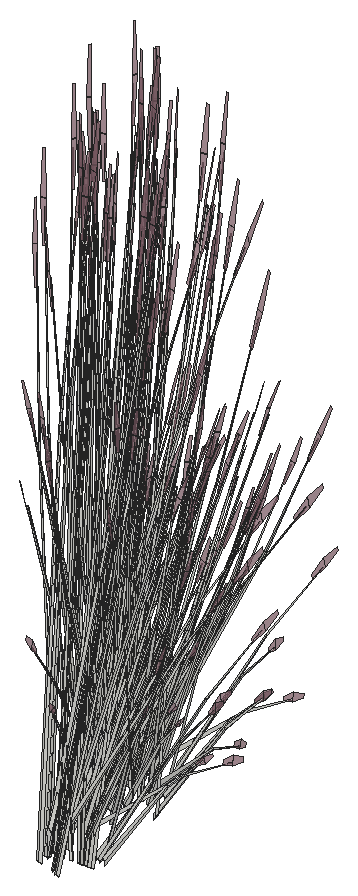
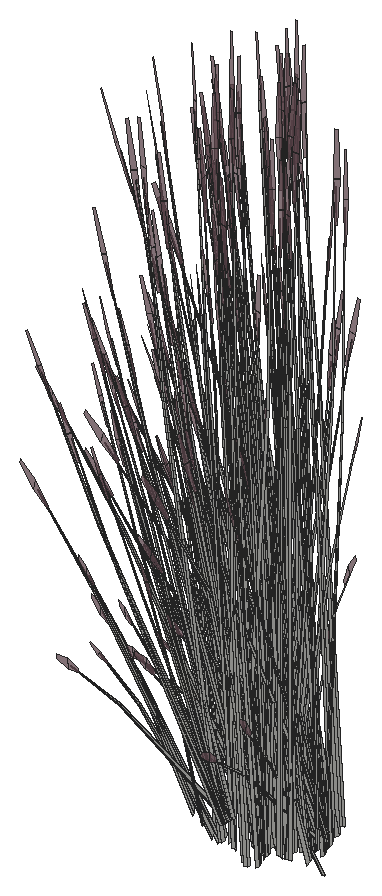
# SketchUp Ruby script. Lengths in inches.
U = 1.inch
M = Sketchup.active_model
def pt(a) = Geom::Point3d.new(a.map { |v| v * U })
def face(e, loops, mat)
  f = e.add_face(loops[0].map { |a| pt(a) })
  loops[1..].each { |l| e.add_face(l.map { |a| pt(a) }).erase! }
  f.material = f.back_material = mat if mat
  f
end
# faces: each face lists its corners as indices into pts; further lists are holes
def faces(e, pts, list, mat = nil) = list.each { |f| face(e, (f[0].is_a?(Array) ? f : [f]).map { |l| l.map { |i| pts[i] } }, mat) }
# xy, xz, yz: faces in a plane at the given z, y or x. An outline is a flat list of corners, or four numbers for a rectangle; further outlines are holes
def ring(l) = l.size == 4 ? [[l[0], l[1]], [l[2], l[1]], [l[2], l[3]], [l[0], l[3]]] : l.each_slice(2).to_a
def flat(e, list, mat, &to3) = list.each { |f| face(e, (f[0].is_a?(Array) ? f : [f]).map { |l| ring(l).map { |u, v| to3.(u, v) } }, mat) }
def xy(e, z, list, mat = nil) = flat(e, list, mat) { |x, y| [x, y, z] }
def xz(e, y, list, mat = nil) = flat(e, list, mat) { |x, z| [x, y, z] }
def yz(e, x, list, mat = nil) = flat(e, list, mat) { |y, z| [x, y, z] }
def lines(e, pts, list) = list.each { |a, b| e.add_line(pt(pts[a]), pt(pts[b])) }
# prism: a flat outline (further loops are holes) pulled along v
def prism(e, loops, v, mat = nil)
  f = face(e, loops, mat); d = Geom::Vector3d.new(v.map { |x| x * U })
  f.pushpull(f.normal.samedirection?(d) ? d.length : -d.length)
end
def box(e, o, s, mat = nil) = prism(e, [[o, [o[0] + s[0], o[1], o[2]], [o[0] + s[0], o[1] + s[1], o[2]], [o[0], o[1] + s[1], o[2]]]], [0, 0, s[2]], mat)
def at(x, y, z, deg = 0) = Geom::Transformation.translation(pt([x, y, z])) * Geom::Transformation.rotation(ORIGIN, Z_AXIS, deg.degrees)
def axes(o, x, y, z) = Geom::Transformation.new([*x, 0, *y, 0, *z, 0, *pt(o).to_a, 1])
def part(name) = M.definitions.add(name)
# library, detail: a bought-in or finely detailed component or shape, given as its bounding box
def library(name, o, s) = part(name).tap { |d| box(d.entities, o, s) }
def detail(e, o, s) = box(e.add_group.entities, o, s)
def put(e, d, t, mat = nil) = e.add_instance(d, t).tap { |i| i.material = mat if mat }
def group(e, t, mat = nil) = e.add_group.tap { |g| g.transformation = t; g.material = mat if mat }.entities
root = M.entities
M.materials.add("LightPink_Translucent").color = [144, 107, 117]
M.materials["LightPink_Translucent"].alpha = 0.75
c1 = part("blade")
p = [[2.15,0.21,22],[0,0.17,0],[0.09,0.45,0],[2.18,0.31,22],[2.29,0.31,22],[0.38,0.45,0],
  [2.48,0.24,33],[2.49,0.24,33],[2.48,0.22,33]]
faces(c1.entities,p,[[0,1,2,3],[4,5,2,3],[6,3,4,7],[8,0,3,6]])
c2 = part("seeds")
p = [[0.3,-0.1,1.38],[-0.01,-0.03,1.59],[-0.01,-0.03,0.03],[0.14,-0.07,-0.07],[0.29,-0.03,3],[0.15,0.01,3.11]]
faces(c2.entities,p,[[0,1,2,3],[1,0,4,5]],"LightPink_Translucent")
c3 = part("blade with seeds")
put(c3.entities,c1,at(0,0,0))
put(c3.entities,c2,axes([2.4,0.25,30.99],[1.5799,-0.05474,1.17369],[-0.12525,1.92788,0.29478],[-0.07173,-0.02425,1.56792]))
put(root,c3,axes([345.62,181.14,6.17],[-0.16657,0.22426,1.71376],[-0.69879,-0.4641,0.13857],[0.31524,-0.28926,0.73262]))
put(root,c3,axes([347.89,180.04,7],[-0.09085,0.04984,1.77383],[-0.89014,-0.16814,-0.16761],[-0.03222,-0.21748,0.31391]))
put(root,c3,axes([345.17,175.54,2.67],[0.90324,-0.43318,-0.29095],[0.60064,0.61207,-0.50002],[0.22285,0.06216,1.59708]))
put(root,c3,axes([348.76,176.68,4.53],[0.74348,0.18202,-0.35414],[-0.21685,0.53102,0.4572],[0.29933,-0.04869,0.87481]))
put(root,c3,axes([347.45,174.39,2.02],[0.83726,0.32623,-0.49651],[-0.50045,0.58498,0],[0.19069,0.0743,1.57504]))
put(root,c3,axes([345.86,176.25,2.21],[1.00089,0,0],[0,0.67548,0],[0,0,1.78407]))
put(root,c3,axes([345.16,179.42,5.06],[0.11476,0.38047,1.1486],[-0.63664,-0.21072,0.84392],[0.06851,-0.19481,0.25299]))
put(root,c3,axes([346.15,174.66,2.47],[-0.96132,0.17317,0.17642],[-0.23737,-0.64447,0.35086],[0.08574,0.0939,1.60407]))
put(root,c3,axes([346.52,181.25,6.97],[-0.64041,-0.4384,-0.51099],[0.67652,-0.38394,-0.3958],[0.09744,-0.22274,0.97773]))
put(root,c3,axes([346.74,176.02,3.875],[-0.37107,0.01478,1.71376],[0.24616,-0.64047,0.13857],[0.5288,0.03961,0.73262]))
put(root,c3,axes([347.22,174.63,2.03],[0.21015,0.56852,-0.30978],[-0.83462,0.16144,0.30978],[0.16826,0.06556,1.38974]))
put(root,c3,axes([348.66,176.9,4.73],[0.32857,0.44488,0.0643],[-0.59916,0.21775,0.50621],[0.26412,-0.04296,0.77189]))
put(root,c3,axes([345.54,175.9,2.38],[-1.13071,-0.13747,0.49198],[0.23011,-0.77639,0.19306],[0.16524,0.07497,1.70813]))
put(root,c3,axes([348.59,176.75,4.73],[-0.25275,0.59491,0.48003],[-0.83094,-0.20343,0.3958],[0.32677,-0.03575,0.9933]))
put(root,c3,axes([345.12,180.59,7.03],[0.88151,0.17057,0.48003],[-0.30143,0.56078,0.3958],[-0.05297,-0.22053,0.9933]))
put(root,c3,axes([344.64,177.82,2.2],[-0.29189,-0.56252,0],[0.83351,-0.19699,0],[0,0,1.54371]))
put(root,c3,axes([347.19,181.48,7.33],[-0.98321,-0.03233,-0.1216],[0.02687,-0.61208,-0.67495],[0.0683,-0.23574,1.02557]))
put(root,c3,axes([347.12,181.08,6.82],[0.60531,-0.34352,-0.35414],[0.573,0.39225,0.4572],[0.08718,-0.19929,0.87481]))
put(root,c3,axes([345.35,180.55,7.02],[0.6592,-0.22175,0.0643],[0.32265,0.40436,0.50621],[-0.06366,-0.17825,0.77189]))
put(root,c3,axes([345.73,177.74,2.18],[0.93921,-0.22138,-0.19198],[0.33003,0.6377,0.00008],[0.10367,-0.02447,1.73897]))
put(root,c3,axes([345.84,176.54,2.21],[0.62448,0.42144,0],[-0.62448,0.42144,0],[0,0,1.69266]))
put(root,c3,axes([347.53,176.35,2.47],[-0.70288,-0.47526,0.17642],[0.70832,-0.46097,0.35086],[-0.07763,0.09706,1.60407]))
put(root,c3,axes([346.23,175.64,2.06],[0.9306,0.10697,-0.62353],[-0.19638,0.65984,-0.16365],[0.27771,0.07995,1.37633]))
put(root,c3,axes([350.34,176.79,2.77],[-0.55274,0.10771,1.1486],[0.26018,-0.44517,0.84392],[0.29323,0.03046,0.25299]))
put(root,c3,axes([345.83,176.04,2.72],[0.43405,-0.58792,0.44739],[0.90188,0.28295,-0.21531],[0,0.13553,1.43643]))
put(root,c3,axes([350.09,178.67,4.71],[-0.08089,-0.05712,1.77383],[0.17695,-0.61228,-0.16761],[0.31864,-0.03912,0.31391]))
put(root,c3,axes([347.88,180.875,3.79],[-0.1339,-0.0514,1.76342],[-0.34394,-0.57425,-0.26939],[0.23202,-0.15583,0.30037]))
put(root,c3,axes([345.67,176.38,2.29],[0,0.75458,-0.05637],[-1.11865,0,0],[0,0.02371,1.79368]))
put(root,c3,axes([345.75,175.85,2.21],[0.53742,0.54764,-0.44739],[-0.81403,0.38564,0.21531],[0.17391,0.06776,1.43643]))
put(root,c3,axes([349.38,178.16,3.93],[-0.17122,-0.54847,-0.03492],[0.80929,-0.12609,-0.15832],[0.169,0.03477,0.52218]))
put(root,c3,axes([347.28,178.15,5.03],[0.0479,-0.66354,-0.1216],[0.90696,0.01814,-0.67495],[0.3493,0.04609,1.02557]))
put(root,c3,axes([348.11,176.37,2.48],[0,-0.65246,0.49651],[1.00089,0,0],[0,0.1486,1.57504]))
put(root,c3,axes([347.12,181.22,7.03],[0.63704,0.44518,0.48003],[-0.67652,0.38394,0.3958],[0.11751,-0.20886,0.9933]))
put(root,c3,axes([346.21,176.18,2.62],[0.83351,-0.19028,0.1448],[0.29189,0.54335,-0.41347],[0,0.11958,1.26744]))
put(root,c3,axes([347.36,181.26,7.02],[0.73517,0.0304,0.0643],[-0.02016,0.45906,0.50621],[0.07693,-0.17585,0.77189]))
put(root,c3,axes([347.14,177.89,5.05],[-0.50902,-0.40851,0.35414],[0.58122,-0.38671,-0.4572],[0.29531,0.05884,0.87481]))
put(root,c3,axes([346.81,181.57,7.34],[-0.60531,0.34352,0.35414],[-0.573,-0.39225,-0.4572],[0.08718,-0.19929,0.87481]))
put(root,c3,axes([347.875,182.5,7.27],[0.4673,-0.51481,-0.71045],[0.81887,0.36587,0.08574],[0.27902,-0.18652,1.00501]))
put(root,c3,axes([349.31,177.5,2.59],[-0.21545,-0.16047,1.43002],[0.28033,-0.53085,-0.30754],[0.43591,0.07191,0.61141]))
put(root,c3,axes([342.82,181,4.67],[-0.55932,-0.6538,0],[0.93577,-0.36461,-0.51607],[0.21313,-0.08304,1.63711]))
put(root,c3,axes([347.85,182.26,6.97],[-0.22982,-0.59576,-0.51099],[0.87033,-0.10422,-0.3958],[0.24941,-0.16002,0.97773]))
put(root,c3,axes([345.45,178.09,2.2],[0.90188,0.29293,0],[-0.43405,0.60866,0],[0,0,1.74954]))
put(root,c3,axes([348.26,182.68,7.33],[-0.82753,-0.35977,-0.1216],[0.47675,-0.52101,-0.67495],[0.2338,-0.18111,1.02557]))
put(root,c3,axes([348.07,177.75,4.72],[0.19191,-0.01103,1.74944],[0.52639,-0.5069,-0.27667],[0.34136,0.06691,0.14031]))
put(root,c3,axes([343.58,180.9,4.3125],[0.83726,-0.32623,-0.49651],[0.50045,0.58498,0],[0.19069,-0.0743,1.57504]))
put(root,c3,axes([348.55,182.02,4.88],[-0.31959,-0.01933,1.43002],[-0.32741,-0.51843,-0.30754],[0.39262,-0.14666,0.61141]))
put(root,c3,axes([350.3,182.53,7],[-0.11685,-0.00496,1.77383],[-0.48522,-0.53096,-0.16761],[0.19486,-0.17458,0.31391]))
put(root,c3,axes([347.33,177.83,4.98],[0.89428,0.01571,-0.71045],[-0.06006,0.66153,0.08574],[0.37886,0.06981,1.00501]))
put(root,c3,axes([344.57,182.23,4.35],[0.60257,-0.49041,-0.62353],[0.74854,0.44469,-0.16365],[0.24146,-0.12234,1.37633]))
put(root,c3,axes([348.92,181.07,5.06],[-0.29798,0.33213,1.1486],[-0.25612,-0.44624,0.84392],[0.24611,-0.11182,0.25299]))
put(root,c3,axes([345.13,177.84,2.29],[0.38895,0.74956,-0.06012],[-1.11135,0.26265,0],[0.01358,0.02618,1.72173]))
put(root,c3,axes([348.79,176.48,2.375],[1.11865,0,0],[0,0.72922,-0.51607],[0,0.16609,1.63711]))
put(root,c3,axes([348.49,182.32,6.82],[0.77872,-0.09325,-0.35414],[0.20563,0.53305,0.4572],[0.22316,-0.14318,0.87481]))
put(root,c3,axes([348.34,176.86,2.2],[-1.1181,-0.00522,-0.04976],[0,-0.72922,0.49943],[-0.03514,0.166,1.58352]))
put(root,c3,axes([345.92,176.22,2.67],[1.00749,0.31132,-0.29095],[-0.48511,0.65709,-0.50002],[0.03166,0.16133,1.59708]))
put(root,c3,axes([347.87,178.1,4.53],[0.50902,0.40851,-0.35414],[-0.58122,0.38671,0.4572],[0.29531,0.05884,0.87481]))
put(root,c3,axes([348.11,176.96,2.03],[-0.62448,0.40708,-0.30978],[-0.62448,-0.40708,0.30978],[0,0.13112,1.38974]))
put(root,c3,axes([343.53,183.09,4.5],[0.43405,-0.58792,-0.44739],[0.90188,0.28295,0.21531],[0,-0.13553,1.43643]))
put(root,c3,axes([347.61,178.26,4.73],[-0.04505,0.49615,0.0643],[-0.68022,-0.0136,0.50621],[0.26056,0.05192,0.77189]))
put(root,c3,axes([343.92,182.8,4.96],[-0.10425,-0.7445,-0.29095],[1.08575,-0.04502,-0.50002],[0.19119,-0.09917,1.59708]))
put(root,c3,axes([345.81,176.71,2.21],[-0.43405,0.58792,-0.44739],[-0.90188,-0.28295,0.21531],[0,0.13553,1.43643]))
put(root,c3,axes([347.67,178.1,4.73],[-0.65964,0.42992,0.48003],[-0.5689,-0.45657,0.3958],[0.30948,0.0793,0.9933]))
put(root,c3,axes([347.86,182.63,7.34],[-0.77872,0.09325,0.35414],[-0.20563,-0.53305,-0.4572],[0.22316,-0.14318,0.87481]))
put(root,c3,axes([343.78,181.15,4.32],[0.83462,0.16144,-0.30978],[-0.21015,0.56852,0.30978],[0.16826,-0.06556,1.38974]))
put(root,c3,axes([345.57,178.59,5.05],[-0.13817,-0.52554,0.35414],[0.78985,-0.13877,-0.4572],[0.21215,0.1506,0.87481]))
put(root,c3,axes([348.54,176.98,2.02],[0,0.65246,-0.49651],[-1.00089,0,0],[0,0.1486,1.57504]))
put(root,c3,axes([346.04,177.05,3.875],[-0.3323,-0.11241,1.71376],[0.68769,-0.4716,0.13857],[0.42861,0.21275,0.73262]))
put(root,c3,axes([346.1,175.57,4.47],[-0.77304,-0.33901,1.38283],[0.81626,-0.52782,0.59665],[0.24941,0.31809,1.33663]))
put(root,c3,axes([348.5625,182.55,7.02],[0.61415,0.2744,0.0643],[-0.35756,0.39076,0.50621],[0.1969,-0.12633,0.77189]))
put(root,c3,axes([348.39,182.43,7.03],[0.22187,0.60049,0.48003],[-0.87033,0.10422,0.3958],[0.25651,-0.14123,0.9933]))
put(root,c3,axes([350.74,183.16,7.01],[0.12414,-0.09938,1.74944],[-0.15889,-0.60963,-0.27667],[0.31148,-0.11559,0.14031]))
put(root,c3,axes([347.27,178.33,2.77],[-0.5037,-0.18761,1.1486],[0.6504,-0.19062,0.84392],[0.17543,0.16147,0.25299]))
put(root,c3,axes([345.5,178.87,5.03],[0.53309,-0.55848,-0.1216],[0.77201,0.32175,-0.67495],[0.26836,0.15779,1.02557]))
put(root,c3,axes([344.0625,183.39,4.73],[1.00799,0.31623,0.24065],[-0.48511,0.65709,0.50002],[0,-0.15147,1.60543]))
put(root,c3,axes([344.8,179.33,4.71],[0.00265,-0.07899,1.77383],[0.76665,-0.34851,-0.16761],[0.2663,0.12439,0.31391]))
put(root,c3,axes([347.41,179.03,1.49],[0.06518,-0.0942,1.76342],[0.82057,-0.27742,-0.26939],[0.24877,0.14358,0.30037]))
put(root,c3,axes([346.33,176.89,2.09],[0.32803,0.59738,-0.69212],[-0.94492,0.21515,-0.18165],[0.03626,0.20229,1.52773]))
put(root,c3,axes([346.13,178.59,4.68],[0.88277,-0.1551,-0.51099],[0.15442,0.58737,-0.3958],[0.23711,0.16832,0.97773]))
put(root,c3,axes([343.74,182.94,5.01],[-0.97146,0.04028,0.44739],[-0.08785,-0.66859,-0.21531],[0.17391,-0.06776,1.43643]))
put(root,c3,axes([343.68,178.68,5.05],[0.2697,-0.50175,0.35414],[0.78684,0.14635,-0.4572],[0.07215,0.20201,0.87481]))
put(root,c3,axes([348.29,184.09,7.33],[-0.45012,-0.59081,-0.1216],[0.79888,-0.29033,-0.67495],[0.33665,-0.07795,1.02557]))
put(root,c3,axes([348.26,183.58,6.97],[0.24236,-0.59349,-0.51099],[0.83094,0.20343,-0.3958],[0.33455,-0.05442,0.97773]))
put(root,c3,axes([346.94,181.16,4.67],[0.55932,-0.6538,0],[0.93577,0.36461,-0.51607],[0.21313,0.08304,1.63711]))
put(root,c3,axes([347.35,179.1875,2.67],[-0.57368,-0.02046,1.0506],[0.37886,-0.43461,0.58006],[0.22663,0.15441,0.8241]))
put(root,c3,axes([343.7,183.1875,4.65],[0.38895,0.72959,0.45755],[-1.11135,0.2537,0.17955],[0.01358,-0.13406,1.58856]))
put(root,c3,axes([349.14,183.75,4.28],[-0.57619,0.0783,1.41583],[-0.09171,-0.62326,0.08104],[0.40356,-0.09434,0.80566]))
put(root,c3,axes([350.19,183.19,4.55],[-0.55463,-0.41721,-0.06488],[0.60744,-0.38228,-0.29416],[0.17212,-0.02691,0.97024]))
put(root,c3,axes([345.7,179.07,4.73],[-0.4066,0.41448,0.0643],[-0.57901,-0.24131,0.50621],[0.18719,0.13288,0.77189]))
put(root,c3,axes([344.74,180.47,5.65],[0.61821,-0.37431,-0.06488],[0.56645,0.40995,-0.29416],[0.03988,0.11616,0.97024]))
put(root,c3,axes([345.1,183.25,4.5],[0,-0.75495,0],[1.11865,0,0],[0,0,1.79456]))
put(root,c3,axes([345.87,178.96,4.73],[-0.88979,0.14973,0.48003],[-0.15442,-0.58737,0.3958],[0.20926,0.17311,0.9933]))
put(root,c3,axes([346.46,181.5,4.77],[-0.83726,-0.32623,0.49651],[0.50045,-0.58498,0],[0.19069,0.0743,1.57504]))
put(root,c3,axes([348.1,183.79,7.27],[0.78611,-0.28816,-0.71045],[0.4381,0.59317,0.08574],[0.37982,-0.06738,1.00501]))
put(root,c3,axes([344.57,182.77,4.65],[-0.74176,0.59212,0.45755],[-0.88124,-0.52269,0.17955],[0.17882,-0.05909,1.58856]))
put(root,c3,axes([345.48,178.13,2.59],[0.01579,-0.21629,1.43002],[0.75442,-0.24159,-0.30754],[0.23289,0.25887,0.61141]))
put(root,c3,axes([343.29,181.8,4.77],[-0.25843,0.64844,0.17642],[-0.9457,-0.1835,0.35086],[0.16336,-0.00316,1.60407]))
put(root,c3,axes([347.98,183.91,7.34],[-0.74348,-0.18202,0.35414],[0.21685,-0.53102,-0.4572],[0.29933,-0.04869,0.87481]))
put(root,c3,axes([343.42,178.89,5.03],[0.87543,-0.30377,-0.1216],[0.4302,0.53915,-0.67495],[0.1155,0.2272,1.02557]))
put(root,c3,axes([342.89,182.32,3.89],[-0.88056,0.26122,1.28929],[-0.28027,-0.74951,0.50096],[0.54072,0.01247,1.46642]))
put(root,c3,axes([345.26,182.52,4.91],[0.17258,-0.58229,0.1448],[0.84319,0.10108,-0.41347],[0.15345,0.05979,1.26744]))
put(root,c3,axes([349.77,183.34,3.79],[-0.04675,-0.09906,1.76342],[0.32428,-0.57943,-0.26939],[0.32711,-0.00833,0.30037]))
put(root,c3,axes([343.58,179.01,1.49],[0.14478,-0.0355,1.76342],[0.8709,0.19542,-0.26939],[0.02547,0.22025,0.30037]))
put(root,c3,axes([344.9,182.67,5.01],[-0.53742,-0.54764,0.44739],[0.81403,-0.38564,-0.21531],[0.17391,0.06776,1.43643]))
put(root,c3,axes([344.17,178.86,4.68],[0.87941,0.16356,-0.51099],[-0.30143,0.56078,-0.3958],[0.08064,0.22578,0.97773]))
put(root,c3,axes([344.67,177.71,3.875],[-0.2045,-0.20949,1.71376],[0.94495,-0.17636,0.13857],[0.21357,0.32887,0.73262]))
put(root,c3,axes([345.17,182.71,4.96],[0.90324,-0.43318,-0.29095],[0.60064,0.61207,-0.50002],[0.22285,0.06216,1.59708]))
put(root,c3,axes([348.76,183.85,6.82],[0.74348,0.18202,-0.35414],[-0.21685,0.53102,0.4572],[0.29933,-0.04869,0.87481]))
put(root,c3,axes([347.45,181.56,4.3125],[0.83726,0.32623,-0.49651],[-0.50045,0.58498,0],[0.19069,0.0743,1.57504]))
put(root,c3,axes([345.86,183.42,4.5],[1.00089,0,0],[0,0.67548,0],[0,0,1.78407]))
put(root,c3,axes([343.77,179.21,4.53],[-0.2697,0.50175,-0.35414],[-0.78684,-0.14635,0.4572],[0.07215,0.20201,0.87481]))
put(root,c3,axes([346.15,181.83,4.77],[-0.96132,0.17317,0.17642],[-0.23737,-0.64447,0.35086],[0.08574,0.0939,1.60407]))
put(root,c3,axes([346.74,183.19,6.17],[-0.37107,0.01478,1.71376],[0.24616,-0.64047,0.13857],[0.5288,0.03961,0.73262]))
put(root,c3,axes([347.22,181.8,4.32],[0.21015,0.56852,-0.30978],[-0.83462,0.16144,0.30978],[0.16826,0.06556,1.38974]))
put(root,c3,axes([348.66,184.07,7.02],[0.32857,0.44488,0.0643],[-0.59916,0.21775,0.50621],[0.26412,-0.04296,0.77189]))
put(root,c3,axes([345.54,183.07,4.67],[-1.13071,-0.13747,0.49198],[0.23011,-0.77639,0.19306],[0.16524,0.07497,1.70813]))
put(root,c3,axes([348.59,183.91,7.03],[-0.25275,0.59491,0.48003],[-0.83094,-0.20343,0.3958],[0.32677,-0.03575,0.9933]))
put(root,c3,axes([344.64,184.99,4.5],[-0.29189,-0.56252,0],[0.83351,-0.19699,0],[0,0,1.54371]))
put(root,c3,axes([343.85,178.76,4.98],[0.42698,0.53052,-0.71045],[-0.87893,0.29566,0.08574],[0.09984,0.25633,1.00501]))
put(root,c3,axes([345.73,184.91,4.48],[0.93921,-0.22138,-0.19198],[0.33003,0.6377,0.00008],[0.10367,-0.02447,1.73897]))
put(root,c3,axes([345.84,183.71,4.51],[0.62448,0.42144,0],[-0.62448,0.42144,0],[0,0,1.69266]))
put(root,c3,axes([343.21,180.1,4.72],[0.1134,0.10507,1.74944],[0.91515,0.04128,-0.27667],[0.09203,0.23172,0.14031]))
put(root,c3,axes([347.53,183.52,4.77],[-0.70288,-0.47526,0.17642],[0.70832,-0.46097,0.35086],[-0.07763,0.09706,1.60407]))
put(root,c3,axes([346.23,182.8,4.35],[0.9306,0.10697,-0.62353],[-0.19638,0.65984,-0.16365],[0.27771,0.07995,1.37633]))
put(root,c3,axes([350.34,183.96,5.06],[-0.55274,0.10771,1.1486],[0.26018,-0.44517,0.84392],[0.29323,0.03046,0.25299]))
put(root,c3,axes([345.83,183.21,5.01],[0.43405,-0.58792,0.44739],[0.90188,0.28295,-0.21531],[0,0.13553,1.43643]))
put(root,c3,axes([350.09,185.84,7],[-0.08089,-0.05712,1.77383],[0.17695,-0.61228,-0.16761],[0.31864,-0.03912,0.31391]))
put(root,c3,axes([345.67,183.55,4.59],[0,0.75458,-0.05637],[-1.11865,0,0],[0,0.02371,1.79368]))
put(root,c3,axes([345.75,183.01,4.5],[0.53742,0.54764,-0.44739],[-0.81403,0.38564,0.21531],[0.17391,0.06776,1.43643]))
put(root,c3,axes([349.38,185.33,6.22],[-0.17122,-0.54847,-0.03492],[0.80929,-0.12609,-0.15832],[0.169,0.03477,0.52218]))
put(root,c3,axes([347.28,185.3125,7.33],[0.0479,-0.66354,-0.1216],[0.90696,0.01814,-0.67495],[0.3493,0.04609,1.02557]))
put(root,c3,axes([348.11,183.54,4.77],[0,-0.65246,0.49651],[1.00089,0,0],[0,0.1486,1.57504]))
put(root,c3,axes([346.21,183.35,4.91],[0.83351,-0.19028,0.1448],[0.29189,0.54335,-0.41347],[0,0.11958,1.26744]))
put(root,c3,axes([347.14,185.05,7.34],[-0.50902,-0.40851,0.35414],[0.58122,-0.38671,-0.4572],[0.29531,0.05884,0.87481]))
put(root,c3,axes([349.31,184.67,4.88],[-0.21545,-0.16047,1.43002],[0.28033,-0.53085,-0.30754],[0.43591,0.07191,0.61141]))
put(root,c3,axes([345.45,185.26,4.5],[0.90188,0.29293,0],[-0.43405,0.60866,0],[0,0,1.74954]))
put(root,c3,axes([348.07,184.92,7.01],[0.19191,-0.01103,1.74944],[0.52639,-0.5069,-0.27667],[0.34136,0.06691,0.14031]))
put(root,c3,axes([347.33,184.99,7.27],[0.89428,0.01571,-0.71045],[-0.06006,0.66153,0.08574],[0.37886,0.06981,1.00501]))
put(root,c3,axes([345.13,185.01,4.58],[0.38895,0.74956,-0.06012],[-1.11135,0.26265,0],[0.01358,0.02618,1.72173]))
put(root,c3,axes([348.79,183.65,4.67],[1.11865,0,0],[0,0.72922,-0.51607],[0,0.16609,1.63711]))
put(root,c3,axes([348.34,184.03,4.49],[-1.1181,-0.00522,-0.04976],[0,-0.72922,0.49943],[-0.03514,0.166,1.58352]))
put(root,c3,axes([345.92,183.39,4.96],[1.00749,0.31132,-0.29095],[-0.48511,0.65709,-0.50002],[0.03166,0.16133,1.59708]))
put(root,c3,axes([347.87,185.27,6.82],[0.50902,0.40851,-0.35414],[-0.58122,0.38671,0.4572],[0.29531,0.05884,0.87481]))
put(root,c3,axes([348.11,184.13,4.32],[-0.62448,0.40708,-0.30978],[-0.62448,-0.40708,0.30978],[0,0.13112,1.38974]))
put(root,c3,axes([347.61,185.42,7.02],[-0.04505,0.49615,0.0643],[-0.68022,-0.0136,0.50621],[0.26056,0.05192,0.77189]))
put(root,c3,axes([345.81,183.88,4.5],[-0.43405,0.58792,-0.44739],[-0.90188,-0.28295,0.21531],[0,0.13553,1.43643]))
